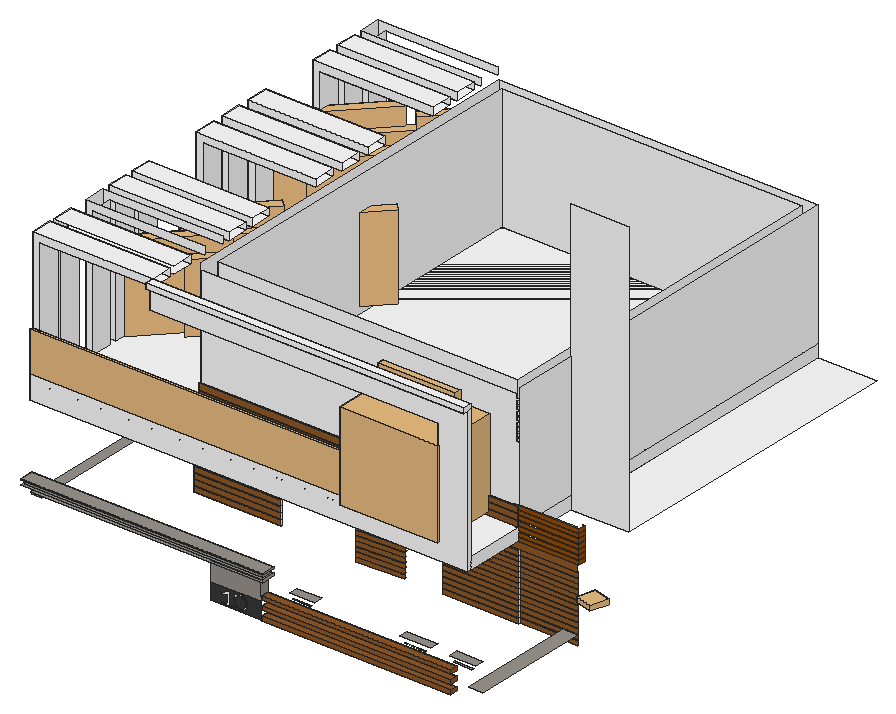
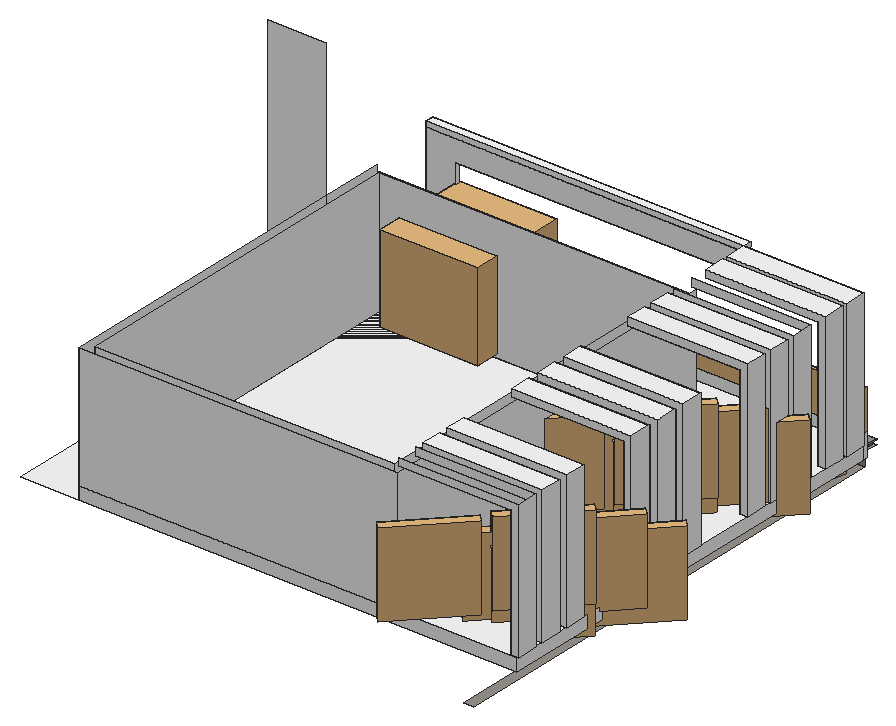
# SketchUp Ruby script. Lengths in inches.
U = 1.inch
M = Sketchup.active_model
def pt(a) = Geom::Point3d.new(a.map { |v| v * U })
def face(e, loops, mat)
  f = e.add_face(loops[0].map { |a| pt(a) })
  loops[1..].each { |l| e.add_face(l.map { |a| pt(a) }).erase! }
  f.material = f.back_material = mat if mat
  f
end
# faces: each face lists its corners as indices into pts; further lists are holes
def faces(e, pts, list, mat = nil) = list.each { |f| face(e, (f[0].is_a?(Array) ? f : [f]).map { |l| l.map { |i| pts[i] } }, mat) }
# xy, xz, yz: faces in a plane at the given z, y or x. An outline is a flat list of corners, or four numbers for a rectangle; further outlines are holes
def ring(l) = l.size == 4 ? [[l[0], l[1]], [l[2], l[1]], [l[2], l[3]], [l[0], l[3]]] : l.each_slice(2).to_a
def flat(e, list, mat, &to3) = list.each { |f| face(e, (f[0].is_a?(Array) ? f : [f]).map { |l| ring(l).map { |u, v| to3.(u, v) } }, mat) }
def xy(e, z, list, mat = nil) = flat(e, list, mat) { |x, y| [x, y, z] }
def xz(e, y, list, mat = nil) = flat(e, list, mat) { |x, z| [x, y, z] }
def yz(e, x, list, mat = nil) = flat(e, list, mat) { |y, z| [x, y, z] }
def lines(e, pts, list) = list.each { |a, b| e.add_line(pt(pts[a]), pt(pts[b])) }
# prism: a flat outline (further loops are holes) pulled along v
def prism(e, loops, v, mat = nil)
  f = face(e, loops, mat); d = Geom::Vector3d.new(v.map { |x| x * U })
  f.pushpull(f.normal.samedirection?(d) ? d.length : -d.length)
end
def box(e, o, s, mat = nil) = prism(e, [[o, [o[0] + s[0], o[1], o[2]], [o[0] + s[0], o[1] + s[1], o[2]], [o[0], o[1] + s[1], o[2]]]], [0, 0, s[2]], mat)
def at(x, y, z, deg = 0) = Geom::Transformation.translation(pt([x, y, z])) * Geom::Transformation.rotation(ORIGIN, Z_AXIS, deg.degrees)
def axes(o, x, y, z) = Geom::Transformation.new([*x, 0, *y, 0, *z, 0, *pt(o).to_a, 1])
def part(name) = M.definitions.add(name)
# library, detail: a bought-in or finely detailed component or shape, given as its bounding box
def library(name, o, s) = part(name).tap { |d| box(d.entities, o, s) }
def detail(e, o, s) = box(e.add_group.entities, o, s)
def put(e, d, t, mat = nil) = e.add_instance(d, t).tap { |i| i.material = mat if mat }
def group(e, t, mat = nil) = e.add_group.tap { |g| g.transformation = t; g.material = mat if mat }.entities
root = M.entities
M.materials.add("[Color C07]").color = [153, 76, 0]
M.materials.add("[Color M00]").color = [255, 255, 255]
M.materials.add("[Color M07]").color = [58, 58, 58]
M.materials.add("[Granite Tile]").color = [155, 148, 143]
M.materials.add("[Translucent Glass Blue]").color = [100, 149, 237]
M.materials["[Translucent Glass Blue]"].alpha = 0.5
M.materials.add("[Wood Floor Parquet]").color = [145, 89, 39]
c1 = part("Group\#32")
box(c1.entities,[0,0,0],[182.46,7.0625,3.98])
c2 = library("ruselia",[-5.83,-15.14,-32.53],[55.24,20.14,57.16])
c3 = library("CM1021-ceilingfixture-VisaLighting.dwg",[51.34,51.34,0],[17.32,17.32,4.91])
c4 = part("CM1021")
put(c4.entities,c3,at(-75.2,7.58,71.26,-15))
put(c4.entities,c3,at(67.3,7.58,71.26,-15))
put(c4.entities,c3,at(180.18,7.58,71.26,-15))
c5 = part("Group\#24")
box(c5.entities,[0,-2.3125,0],[173.47,2.3125,5.79])
c6 = library("Glass+Door+1800+x+2400",[-92.74,-2.96,0],[74.8,10.14,98.43])
c7 = part("Group\#17")
box(c7.entities,[0,-2.125,0],[58.6875,4.9375,2.3125])
c8 = library("Skt_BoxwoodBall_13",[-7.4,-7.46,-2.06],[14.58,14.83,12.98])
c9 = library("Glass railing panel",[0.75,0.33,0],[60,3.22,44.35])
xy(root,48.99,[[491.52,212.5,564.8125,213.625]],"[Color M00]")
xy(root,49.18,[[410.51,209.22,410.4,211.4,455.45,213.78,455.57,211.6]],"[Color M00]")
xy(root,52.66,[[252.1,212.375,336.02,213.625]],"[Color M00]")
xy(root,53.16,[[491.52,212.5,564.8125,213.625]],"[Color M00]")
xy(root,53.35,[[252.1,212.375,336.02,213.625]],"[Color M00]")
xy(root,53.41,[[410.51,209.22,455.57,211.6,455.45,213.78,410.4,211.4]],"[Color M00]")
xy(root,53.8,[[410.51,209.22,410.4,211.4,455.45,213.78,455.57,211.6]],"[Color M00]")
xy(root,54.18,[[491.52,212.5,564.8125,213.625]],"[Color M00]")
xy(root,58.04,[[410.51,209.22,455.57,211.6,455.45,213.78,410.4,211.4]],"[Color M00]")
xy(root,58.35,[[491.52,212.5,564.8125,213.625]],"[Color M00]")
xy(root,58.41,[[252.1,212.375,336.02,213.625]],"[Color M00]")
xy(root,58.61,[[410.51,209.22,410.4,211.4,455.45,213.78,455.57,211.6]],"[Color M00]")
xy(root,58.6875,[[607.56,99.5625,620.89,213.625]],"[Granite Tile]")
xy(root,58.91,[[252.1,212.375,336.02,213.625]],"[Color M00]")
xy(root,59.36,[[491.52,212.5,564.8125,213.625]],"[Color M00]")
xy(root,62.85,[[410.51,209.22,455.57,211.6,455.45,213.78,410.4,211.4]],"[Color M00]")
xy(root,63.24,[[410.51,209.22,410.4,211.4,455.45,213.78,455.57,211.6]],"[Color M00]")
xy(root,63.54,[[491.52,212.5,564.8125,213.625]],"[Color M00]")
xy(root,63.97,[[252.1,212.375,336.02,213.625]],"[Color M00]")
xy(root,64.36,[[491.52,212.5,564.8125,213.625]],"[Color M00]")
xy(root,64.6,[[252.1,212.375,336.02,213.625]],"[Color M00]")
xy(root,67.48,[[410.51,209.22,455.57,211.6,455.45,213.78,410.4,211.4]],"[Color M00]")
xy(root,67.93,[[410.51,209.22,410.4,211.4,455.45,213.78,455.57,211.6]],"[Color M00]")
xy(root,68.54,[[491.52,212.5,564.8125,213.625]],"[Color M00]")
xy(root,69.36,[[491.52,212.5,564.8125,213.625]],"[Color M00]")
xy(root,69.66,[[252.1,212.375,336.02,213.625]],"[Color M00]")
xy(root,70.28,[[252.1,212.375,336.02,213.625]],"[Color M00]")
xy(root,72.16,[[410.51,209.22,455.57,211.6,455.45,213.78,410.4,211.4]],"[Color M00]")
xy(root,72.78,[[410.62,209.22,410.5,211.41,455.55,213.79,455.67,211.6]],"[Color M00]")
xy(root,73.54,[[491.52,212.5,564.8125,213.625]],"[Color M00]")
xy(root,74.43,[[491.52,212.5,564.8125,213.625]],"[Color M00]")
xy(root,75.35,[[252.1,212.375,336.02,213.625]],"[Color M00]")
xy(root,75.6875,[[183.25,102.22,193.4375,573.625]],"[Granite Tile]")
xy(root,75.78,[[252.1,212.375,336.02,213.625]],"[Color M00]")
xy(root,77.01,[[410.62,209.22,455.67,211.6,455.55,213.79,410.5,211.41]],"[Color M00]")
xy(root,77.25,[[410.74,209,410.63,211.18,455.68,213.57,455.8,211.38]],"[Color M00]")
xy(root,78.6,[[491.52,212.5,564.8125,213.625]],"[Color M00]")
xy(root,79.18,[[491.52,212.5,564.8125,213.625]],"[Color M00]")
xy(root,80.75,[[551.82,91.25,572.14,91.8125]],"[Granite Tile]")
xy(root,80.85,[[252.1,212.375,336.02,213.625]],"[Color M00]")
xy(root,80.85,[[598.93,91.25,617.05,93]],"[Granite Tile]")
xy(root,80.89,[[444.42,91.25,461.86,91.8125]],"[Granite Tile]")
xy(root,81.47,[[252.1,212.375,336.02,213.625]],"[Color M00]")
xy(root,81.49,[[410.74,209,455.8,211.38,455.68,213.57,410.63,211.18]],"[Color M00]")
xy(root,81.9375,[[410.74,209,410.63,211.18,455.68,213.57,455.8,211.38]],"[Color M00]")
xy(root,83.35,[[491.52,212.5,564.8125,213.625]],"[Color M00]")
xy(root,83.93,[[491.52,212.5,564.8125,213.625]],"[Color M00]")
xy(root,85.375,[[440.87,91.25,465.26,99.5625],[547.3,91.25,577.46,99.5625],[595.47,91.25,620.89,99.5625]],"[Granite Tile]")
xy(root,86.18,[[410.74,209,455.8,211.38,455.68,213.57,410.63,211.18]],"[Color M00]")
xy(root,86.53,[[252.1,212.375,336.02,213.625]],"[Color M00]")
xy(root,86.6875,[[410.74,209,410.63,211.18,455.68,213.57,455.8,211.38]],"[Color M00]")
xy(root,86.92,[[193.4375,88.8125,417,102.22]],"[Granite Tile]")
xy(root,86.9375,[[364.82,91.25,413.01,99.5625]],"[Granite Tile]")
xy(root,87.58,[[252.1,212.375,336.02,213.625]],"[Color M00]")
xy(root,88.1,[[491.52,212.5,564.8125,213.625]],"[Color M00]")
xy(root,88.68,[[491.52,212.5,564.8125,213.625]],"[Color M00]")
xy(root,89.375,[[[183.25,88.8125,417,102.22],[185.6,91.54,415.04,100.36]]],"[Granite Tile]")
xy(root,90.93,[[410.74,209,455.8,211.38,455.68,213.57,410.63,211.18]],"[Color M00]")
xy(root,91.3125,[[410.74,209,410.63,211.18,455.68,213.57,455.8,211.38]],"[Color M00]")
xy(root,92.64,[[252.1,212.375,336.02,213.625]],"[Color M00]")
xy(root,92.85,[[491.52,212.5,564.8125,213.625]],"[Color M00]")
xy(root,93,[[183.25,88.8125,417,91.54],[183.25,91.54,185.6,102.22],[415.04,91.54,417,100.36],[185.6,100.36,417,102.22]],"[Granite Tile]")
xy(root,93.36,[[491.52,212.5,564.8125,213.625]],"[Color M00]")
xy(root,93.64,[[252.1,212.375,336.02,213.625]],"[Color M00]")
xy(root,94.5625,[[183.25,88.8125,417,102.22]],"[Granite Tile]")
xy(root,95.55,[[410.74,209,455.8,211.38,455.68,213.57,410.63,211.18]],"[Color M00]")
xy(root,96.875,[[410.74,209,410.63,211.18,455.68,213.57,455.8,211.38]],"[Color M00]")
xy(root,97.54,[[491.52,212.5,564.8125,213.625]],"[Color M00]")
xy(root,97.99,[[491.52,212.5,564.8125,213.625]],"[Color M00]")
xy(root,98.7,[[252.1,212.375,336.02,213.625]],"[Color M00]")
xy(root,99.83,[[252.1,212.375,336.02,213.625]],"[Color M00]")
xy(root,101.11,[[410.74,209,455.8,211.38,455.68,213.57,410.63,211.18]],"[Color M00]")
xy(root,102,[[410.74,209,410.63,211.18,455.68,213.57,455.8,211.38]],"[Color M00]")
xy(root,102.16,[[491.52,212.5,564.8125,213.625]],"[Color M00]")
xy(root,102.82,[[491.52,212.5,564.8125,213.625]],"[Color M00]")
xy(root,104.89,[[252.1,212.375,336.02,213.625]],"[Color M00]")
xy(root,106.14,[[252.1,212.375,336.02,213.625]],"[Color M00]")
xy(root,106.24,[[410.74,209,455.8,211.38,455.68,213.57,410.63,211.18]],"[Color M00]")
xy(root,106.875,[[410.74,209,410.63,211.18,455.68,213.57,455.8,211.38]],"[Color M00]")
xy(root,106.99,[[491.52,212.5,564.8125,213.625]],"[Color M00]")
xy(root,107.57,[[491.52,212.5,564.8125,213.625]],"[Color M00]")
xy(root,111.11,[[410.74,209,455.8,211.38,455.68,213.57,410.63,211.18]],"[Color M00]")
xy(root,111.2,[[252.1,212.375,336.02,213.625]],"[Color M00]")
xy(root,111.74,[[491.52,212.5,564.8125,213.625]],"[Color M00]")
xy(root,113.1,[[252.1,212.5,620.9375,213.625]],"[Color M00]")
xy(root,120,[[141.8125,151.875,564.8125,155.5],[252.1,212.5,620.9375,213.625],[564.8125,275.23,620.9375,573.625]],"[Color M00]")
xy(root,120.2,[[561.375,211.8125,561.375,213.625,622.25,213.625,622.25,218.625,623.5625,218.625,623.5625,211.8125]],"[Color M00]")
xy(root,123.76,[[561.375,211.8125,623.5625,211.8125,623.5625,218.625,622.25,218.625,622.25,213.625,561.375,213.625]],"[Color M00]")
xy(root,124.89,[[561.375,211.8125,561.375,213.625,622.25,213.625,622.25,218.625,623.5625,218.625,623.5625,211.8125]],"[Color M00]")
xy(root,128.45,[[561.375,211.8125,623.5625,211.8125,623.5625,218.625,622.25,218.625,622.25,213.625,561.375,213.625]],"[Color M00]")
xy(root,129.65,[[561.375,211.8125,561.375,213.625,622.25,213.625,622.25,218.625,623.5625,218.625,623.5625,211.8125]],"[Color M00]")
xy(root,132,[[[257.3125,213.625,564.8125,573.625],[266.75,222.625,555.8125,564.625]],[141.8125,219.03,149.03,239.92],[266.75,222.625,555.8125,564.625]],"[Color M00]")
xy(root,133.21,[[561.375,211.8125,623.5625,211.8125,623.5625,218.625,622.25,218.625,622.25,213.625,561.375,213.625]],"[Color M00]")
xy(root,134.4,[[561.375,211.8125,561.375,213.625,622.25,213.625,622.25,218.625,623.5625,218.625,623.5625,211.8125]],"[Color M00]")
xy(root,137.96,[[561.375,211.8125,623.5625,211.8125,623.5625,218.625,622.25,218.625,622.25,213.625,561.375,213.625]],"[Color M00]")
xy(root,139.15,[[561.375,211.8125,561.375,213.625,622.25,213.625,622.25,218.625,623.5625,218.625,623.5625,211.8125]],"[Color M00]")
xy(root,142.37,[[141.8125,151.875,535.19,155.5]],"[Color M00]")
xy(root,142.71,[[561.375,211.8125,623.5625,211.8125,623.5625,218.625,622.25,218.625,622.25,213.625,561.375,213.625]],"[Color M00]")
xy(root,143.59,[[561.375,211.8125,561.375,213.625,622.25,213.625,622.25,218.625,623.5625,218.625,623.5625,211.8125]],"[Color M00]")
xy(root,147.15,[[561.375,211.8125,623.5625,211.8125,623.5625,218.625,622.25,218.625,622.25,213.625,561.375,213.625]],"[Color M00]")
xy(root,147.77,[[561.375,211.8125,561.375,213.625,622.25,213.625,622.25,218.625,623.5625,218.625,623.5625,211.8125]],"[Color M00]")
xy(root,238.5625,[[257.3125,151.875,535.19,155.5]],"[Color M00]")
xy(root,256.75,[[149.03,155.5,257.3125,176.39],[149.03,180.8125,257.3125,201.7],[149.03,247.28,257.3125,268.17],[149.03,274.72,257.3125,295.61],[149.03,352.5625,257.3125,373.45],
  [149.03,383.5,257.3125,404.39],[149.03,415.3125,257.3125,436.2],[149.03,492.9375,257.3125,513.83],[149.03,522.625,257.3125,543.51]],"[Color M00]")
xy(root,259.26,[[257.3125,146.9375,564.8125,151.875],[257.3125,151.875,564.8125,155.5]],"[Color M00]")
xy(root,264,[[257.3125,146.9375,564.8125,155.5],[141.8125,155.5,257.3125,176.39],[141.8125,180.8125,257.3125,201.7],[141.8125,247.28,257.3125,268.17],[141.8125,274.72,257.3125,295.61],
  [141.8125,352.5625,257.3125,373.45],[141.8125,383.5,257.3125,404.39],[141.8125,415.3125,257.3125,436.2],[141.8125,492.9375,257.3125,513.83],[141.8125,522.625,257.3125,543.51]],"[Color M00]")
xz(root,88.8125,[[183.25,93,417,94.5625]],"[Granite Tile]")
xz(root,91.25,[[[393.28,53.49,395.01,53.64,396.63,54.23,398.05,55.22,399.16,56.54,399.9,58.11,400.2,59.81,400.05,61.53,399.47,63.16,398.48,64.58,397.15,65.69,395.59,66.43,393.89,66.73,392.16,66.58,390.54,65.99,389.12,65,388,63.68,387.27,62.12,386.97,60.41,387.11,58.69,387.7,57.0625,388.69,55.64,390.01,54.53,391.58,53.8],[393.58,54.86,392.23,55.04,390.96,55.5625,389.87,56.4,389.04,57.49,388.51,58.75,388.33,60.11,388.51,61.47,389.04,62.74,389.87,63.82,390.96,64.66,392.23,65.18,393.58,65.36,394.94,65.18,396.21,64.66,397.3,63.82,398.13,62.74,398.66,61.47,398.83,60.11,398.66,58.75,398.13,57.49,397.3,56.4,396.21,55.5625,394.94,55.04]],[375.79,53.62,387.87,53.62,387.87,54.43,382.16,54.43,382.16,66.03,375.79,62.58,376.9,61.57,380.9375,63.7,380.9375,54.43,375.79,54.43]],"[Color M00]")
xz(root,91.25,[[[364.82,52.49,413.01,68.13],[393.28,53.49,391.58,53.8,390.01,54.53,388.69,55.64,387.7,57.0625,387.11,58.69,386.97,60.41,387.27,62.12,388,63.68,389.12,65,390.54,65.99,392.16,66.58,393.89,66.73,395.59,66.43,397.15,65.69,398.48,64.58,399.47,63.16,400.05,61.53,400.2,59.81,399.9,58.11,399.16,56.54,398.05,55.22,396.63,54.23,395.01,53.64],[375.79,53.62,375.79,54.43,380.9375,54.43,380.9375,63.7,376.9,61.57,375.79,62.58,382.16,66.03,382.16,54.43,387.87,54.43,387.87,53.62]],[393.58,54.86,394.94,55.04,396.21,55.5625,397.3,56.4,398.13,57.49,398.66,58.75,398.83,60.11,398.66,61.47,398.13,62.74,397.3,63.82,396.21,64.66,394.94,65.18,393.58,65.36,392.23,65.18,390.96,64.66,389.87,63.82,389.04,62.74,388.51,61.47,388.33,60.11,388.51,58.75,389.04,57.49,389.87,56.4,390.96,55.5625,392.23,55.04]],"[Color M07]")
xz(root,91.25,[[364.82,68.13,413.01,86.9375]],"[Granite Tile]")
xz(root,91.54,[[185.6,89.375,415.04,93]],"[Granite Tile]")
xz(root,100.36,[[185.6,89.375,415.04,93]],"[Granite Tile]")
xz(root,102.22,[[183.25,75.6875,193.4375,75.6875,193.4375,86.92,417,86.92,417,89.375,183.25,89.375],[183.25,93,417,94.5625]],"[Granite Tile]")
xz(root,146.9375,[[257.3125,259.26,564.8125,264]],"[Color M00]")
xz(root,151.875,[[141.8125,120,564.8125,120,564.8125,259.26,257.3125,259.26,257.3125,238.5625,535.19,238.5625,535.19,142.37,141.8125,142.37]],"[Color M00]")
xz(root,155.5,[[141.8125,120,141.8125,132,149.03,132,149.03,142.37,535.19,142.37,535.19,238.5625,257.3125,238.5625,257.3125,259.26,564.8125,259.26,564.8125,120],[141.8125,132,149.03,142.37],[141.8125,142.37,149.03,142.37,149.03,256.75,257.3125,256.75,257.3125,264,141.8125,264],[257.3125,259.26,564.8125,264]],"[Color M00]")
xz(root,176.39,[[141.8125,132,141.8125,264,257.3125,264,257.3125,256.75,149.03,256.75,149.03,132]],"[Color M00]")
xz(root,180.8125,[[141.8125,132,149.03,142.37]],"[Color M00]")
xz(root,201.7,[[141.8125,132,141.8125,264,257.3125,264,257.3125,256.75,149.03,256.75,149.03,132]],"[Color M00]")
xz(root,211.8125,[[561.375,120.2,623.5625,123.76],[561.375,124.89,623.5625,128.45],[561.375,129.65,623.5625,133.21],[561.375,134.4,623.5625,137.96],[561.375,139.15,623.5625,142.71],
  [561.375,143.59,623.5625,147.15],[561.375,147.77,623.5625,151.34]],"[Color C07]")
xz(root,212.375,[[252.1,53.35,336.02,58.41],[252.1,58.91,336.02,63.97],[252.1,64.6,336.02,69.66],[252.1,70.28,336.02,75.35],[252.1,75.78,336.02,80.85],
  [252.1,81.47,336.02,86.53],[252.1,87.58,336.02,92.64],[252.1,93.64,336.02,98.7],[252.1,99.83,336.02,104.89],[252.1,106.14,336.02,111.2]],"[Wood Floor Parquet]")
xz(root,212.5,[[491.52,48.99,564.8125,53.16],[491.52,54.18,564.8125,58.35],[491.52,59.36,564.8125,63.54],[491.52,64.36,564.8125,68.54],[491.52,69.36,564.8125,73.54],
  [491.52,74.43,564.8125,78.6],[491.52,79.18,564.8125,83.35],[491.52,83.93,564.8125,88.1],[491.52,88.68,564.8125,92.85],[491.52,93.36,564.8125,97.54],
  [491.52,97.99,564.8125,102.16],[491.52,102.82,564.8125,106.99],[491.52,107.57,564.8125,111.74],[252.1,113.1,620.9375,120]],"[Wood Floor Parquet]")
xz(root,213.625,[[252.1,53.35,336.02,58.41],[252.1,58.91,336.02,63.97],[252.1,64.6,336.02,69.66],[252.1,70.28,336.02,75.35],[252.1,75.78,336.02,80.85],
  [252.1,81.47,336.02,86.53],[252.1,87.58,336.02,92.64],[252.1,93.64,336.02,98.7],[252.1,99.83,336.02,104.89],[252.1,106.14,336.02,111.2],
  [491.52,107.57,564.8125,111.74],[257.3125,132,564.8125,132,564.8125,204.71,561.375,204.71,561.375,208.27,564.8125,208.27,564.8125,209.21,561.375,209.21,561.375,212.77,564.8125,212.77,564.8125,213.84,561.375,213.84,561.375,217.4,564.8125,217.4,564.8125,218.15,561.375,218.15,561.375,221.71,564.8125,221.71,564.8125,222.96,561.375,222.96,561.375,226.52,564.8125,226.52,564.8125,227.46,561.375,227.46,561.375,231.02,564.8125,231.02,564.8125,232.46,561.375,232.46,561.375,236.02,564.8125,236.02,564.8125,237.27,561.375,237.27,561.375,240.84,564.8125,240.84,564.8125,242.46,561.375,242.46,561.375,246.02,564.8125,246.02,564.8125,246.21,257.3125,246.21]],"[Color M00]")
xz(root,213.625,[[607.56,58.35,620.89,58.6875]],"[Granite Tile]")
xz(root,213.625,[[564.8125,120,620.9375,120.2],[564.8125,120.2,620.9375,123.76],[564.8125,123.76,620.9375,124.89],[564.8125,124.89,620.9375,128.45],[564.8125,128.45,620.9375,129.65],
  [564.8125,129.65,620.9375,133.21],[564.8125,133.21,620.9375,134.4],[564.8125,134.4,620.9375,137.96],[564.8125,137.96,620.9375,139.15],[564.8125,139.15,620.9375,142.71],
  [564.8125,142.71,620.9375,143.59],[564.8125,143.59,620.9375,147.15],[564.8125,147.15,620.9375,147.77],[564.8125,147.77,620.9375,151.34]],"[Translucent Glass Blue]")
xz(root,213.625,[[564.8125,48.99,607.56,53.16],[607.56,48.99,620.89,53.16],[620.89,48.99,620.9375,53.16],[607.56,53.16,620.89,54.18],[620.89,53.16,620.9375,54.18],
  [564.8125,54.18,607.56,58.35],[607.56,54.18,620.89,58.35],[620.89,54.18,620.9375,58.35],[564.8125,59.36,620.9375,63.54],[564.8125,64.36,620.9375,68.54],
  [564.8125,69.36,620.9375,73.54],[564.8125,74.43,620.9375,78.6],[564.8125,79.18,620.9375,83.35],[564.8125,83.93,620.9375,88.1],[564.8125,88.68,620.9375,92.85],
  [564.8125,93.36,620.9375,97.54],[564.8125,97.99,620.9375,102.16],[564.8125,102.82,620.9375,106.99],[564.8125,107.57,620.9375,111.74]],"[Wood Floor Parquet]")
xz(root,218.625,[[622.25,120.2,623.5625,123.76],[622.25,124.89,623.5625,128.45],[622.25,129.65,623.5625,133.21],[622.25,134.4,623.5625,137.96],[622.25,139.15,623.5625,142.71],
  [622.25,143.59,623.5625,147.15],[622.25,147.77,623.5625,151.34]],"[Color M00]")
xz(root,219.03,[[141.8125,132,149.03,132,149.03,256.75,257.3125,256.75,257.3125,264,141.8125,264]],"[Color M00]")
xz(root,222.625,[[266.75,132,555.8125,252]],"[Color M00]")
xz(root,239.92,[[141.8125,132,141.8125,264,257.3125,264,257.3125,256.75,149.03,256.75,149.03,132]],"[Color M00]")
xz(root,247.28,[[141.8125,132,149.03,132,149.03,256.75,257.3125,256.75,257.3125,264,141.8125,264]],"[Color M00]")
xz(root,268.17,[[141.8125,132,141.8125,264,257.3125,264,257.3125,256.75,149.03,256.75,149.03,132]],"[Color M00]")
xz(root,274.72,[[141.8125,132,149.03,132,149.03,256.75,257.3125,256.75,257.3125,264,141.8125,264]],"[Color M00]")
xz(root,275.23,[[564.8125,120,620.9375,384]],"[Color M00]")
xz(root,295.61,[[141.8125,132,141.8125,264,257.3125,264,257.3125,256.75,149.03,256.75,149.03,132]],"[Color M00]")
xz(root,352.5625,[[141.8125,132,149.03,132,149.03,256.75,257.3125,256.75,257.3125,264,141.8125,264]],"[Color M00]")
xz(root,373.45,[[141.8125,132,141.8125,264,257.3125,264,257.3125,256.75,149.03,256.75,149.03,132]],"[Color M00]")
xz(root,383.5,[[141.8125,132,149.03,132,149.03,256.75,257.3125,256.75,257.3125,264,141.8125,264]],"[Color M00]")
xz(root,404.39,[[141.8125,132,141.8125,264,257.3125,264,257.3125,256.75,149.03,256.75,149.03,132]],"[Color M00]")
xz(root,415.3125,[[141.8125,132,149.03,132,149.03,256.75,257.3125,256.75,257.3125,264,141.8125,264]],"[Color M00]")
xz(root,436.2,[[141.8125,132,141.8125,264,257.3125,264,257.3125,256.75,149.03,256.75,149.03,132]],"[Color M00]")
xz(root,492.9375,[[141.8125,132,149.03,132,149.03,256.75,257.3125,256.75,257.3125,264,141.8125,264]],"[Color M00]")
xz(root,513.83,[[141.8125,132,141.8125,264,257.3125,264,257.3125,256.75,149.03,256.75,149.03,132]],"[Color M00]")
xz(root,522.625,[[141.8125,132,149.03,132,149.03,256.75,257.3125,256.75,257.3125,264,141.8125,264]],"[Color M00]")
xz(root,543.51,[[141.8125,132,141.8125,264,257.3125,264,257.3125,256.75,149.03,256.75,149.03,132]],"[Color M00]")
xz(root,551.125,[[141.8125,132,149.03,132,149.03,256.75,257.3125,256.75,257.3125,264,141.8125,264]],"[Color M00]")
xz(root,564.625,[[266.75,132,555.8125,252]],"[Color M00]")
xz(root,572.01,[[141.8125,132,141.8125,264,257.3125,264,257.3125,256.75,149.03,256.75,149.03,132]],"[Color M00]")
xz(root,573.625,[[257.3125,132,564.8125,252]],"[Color M00]")
yz(root,141.8125,[[151.875,120,155.5,142.37],[155.5,132,176.39,264],[180.8125,132,201.7,264],[219.03,132,239.92,264],[247.28,132,268.17,264],
  [274.72,132,295.61,264],[352.5625,132,373.45,264],[383.5,132,404.39,264],[415.3125,132,436.2,264],[492.9375,132,513.83,264],
  [522.625,132,543.51,264],[551.125,132,572.01,264]],"[Color M00]")
yz(root,149.03,[[155.5,132,176.39,256.75],[180.8125,132,201.7,256.75],[219.03,132,239.92,256.75],[247.28,132,268.17,256.75],[274.72,132,295.61,256.75],
  [352.5625,132,373.45,256.75],[383.5,132,404.39,256.75],[415.3125,132,436.2,256.75],[492.9375,132,513.83,256.75],[522.625,132,543.51,256.75],
  [551.125,132,572.01,256.75]],"[Color M00]")
yz(root,183.25,[[88.8125,93,102.22,94.5625]],"[Granite Tile]")
yz(root,185.6,[[91.54,89.375,100.36,93]],"[Granite Tile]")
yz(root,252.1,[[212.375,53.35,213.625,58.41],[212.375,58.91,213.625,63.97],[212.375,64.6,213.625,69.66],[212.375,70.28,213.625,75.35],[212.375,75.78,213.625,80.85],
  [212.375,81.47,213.625,86.53],[212.375,87.58,213.625,92.64],[212.375,93.64,213.625,98.7],[212.375,99.83,213.625,104.89],[212.375,106.14,213.625,111.2]],"[Color M00]")
yz(root,257.3125,[[213.625,132,573.625,252],[151.875,238.5625,155.5,259.26],[146.9375,259.26,155.5,264]],"[Color M00]")
yz(root,266.75,[[222.625,132,564.625,252]],"[Color M00]")
yz(root,336.02,[[212.375,53.35,213.625,58.41],[212.375,58.91,213.625,63.97],[212.375,64.6,213.625,69.66],[212.375,70.28,213.625,75.35],[212.375,75.78,213.625,80.85],
  [212.375,81.47,213.625,86.53],[212.375,87.58,213.625,92.64],[212.375,93.64,213.625,98.7],[212.375,99.83,213.625,104.89],[212.375,106.14,213.625,111.2]],"[Color M00]")
yz(root,413.01,[[91.25,72.61,99.5625,86.9375]],"[Granite Tile]")
yz(root,415.04,[[91.54,89.375,100.36,93]],"[Granite Tile]")
yz(root,417,[[88.8125,86.92,102.22,89.375],[88.8125,93,102.22,94.5625]],"[Granite Tile]")
yz(root,491.52,[[212.5,107.57,213.625,111.74]],"[Color M00]")
yz(root,535.19,[[151.875,142.37,155.5,238.5625]],"[Color M00]")
yz(root,555.8125,[[222.625,132,564.625,252]],"[Color M00]")
yz(root,564.8125,[[212.5,48.99,213.625,53.16],[212.5,54.18,213.625,58.35],[212.5,59.36,213.625,63.54],[212.5,64.36,213.625,68.54],[212.5,69.36,213.625,73.54],
  [212.5,74.43,213.625,78.6],[212.5,79.18,213.625,83.35],[212.5,83.93,213.625,88.1],[212.5,88.68,213.625,92.85],[212.5,93.36,213.625,97.54],
  [212.5,97.99,213.625,102.16],[212.5,102.82,213.625,106.99],[212.5,107.57,213.625,111.74],[151.875,120,155.5,259.26],[213.625,120,275.23,132],
  [213.625,132,275.23,252],[275.23,132,573.625,252],[146.9375,259.26,155.5,264]],"[Color M00]")
yz(root,623.5625,[[211.8125,120.2,218.625,123.76],[211.8125,124.89,218.625,128.45],[211.8125,129.65,218.625,133.21],[211.8125,134.4,218.625,137.96],[211.8125,139.15,218.625,142.71],
  [211.8125,143.59,218.625,147.15],[211.8125,147.77,218.625,151.34]],"[Color C07]")
p = [[410.51,209.22,49.18],[455.57,211.6,49.18],[455.57,211.6,53.41],[410.51,209.22,53.41],[410.51,209.22,53.8],[455.57,211.6,53.8],
  [455.57,211.6,58.04],[410.51,209.22,58.04],[410.51,209.22,58.61],[455.57,211.6,58.61],[455.57,211.6,62.85],[410.51,209.22,62.85],
  [410.51,209.22,63.24],[455.57,211.6,63.24],[455.57,211.6,67.48],[410.51,209.22,67.48],[410.51,209.22,67.93],[455.57,211.6,67.93],
  [455.57,211.6,72.16],[410.51,209.22,72.16],[410.62,209.22,72.78],[455.67,211.6,72.78],[455.67,211.6,77.01],[410.62,209.22,77.01],
  [410.74,209,77.25],[455.8,211.38,77.25],[455.8,211.38,81.49],[410.74,209,81.49],[410.74,209,81.9375],[455.8,211.38,81.9375],
  [455.8,211.38,86.18],[410.74,209,86.18],[410.74,209,86.6875],[455.8,211.38,86.6875],[455.8,211.38,90.93],[410.74,209,90.93],
  [410.74,209,91.3125],[455.8,211.38,91.3125],[455.8,211.38,95.55],[410.74,209,95.55],[410.74,209,96.875],[455.8,211.38,96.875],
  [455.8,211.38,101.11],[410.74,209,101.11],[410.74,209,102],[455.8,211.38,102],[455.8,211.38,106.24],[410.74,209,106.24],
  [410.63,211.18,111.11],[410.63,211.18,106.875],[410.74,209,106.875],[410.74,209,111.11],[455.8,211.38,106.875],[455.8,211.38,111.11],
  [455.68,213.57,106.875],[455.68,213.57,111.11]]
faces(root,p,[[0,1,2,3],[4,5,6,7],[8,9,10,11],[12,13,14,15],[16,17,18,19],[20,21,22,23],[24,25,26,27],[28,29,30,31],
  [32,33,34,35],[36,37,38,39],[40,41,42,43],[44,45,46,47],[50,52,53,51]],"[Wood Floor Parquet]")
faces(root,p,[[48,49,50,51],[54,49,48,55],[54,55,53,52]],"[Color M00]")
put(root,c1,at(413.01,92.5,50.94),"[Wood Floor Parquet]")
put(root,c1,at(413.01,92.5,59.75),"[Wood Floor Parquet]")
put(root,c1,at(413.01,92.5,68.63),"[Wood Floor Parquet]")
put(root,c2,axes([201.14,521.4,160.65],[-0.97449,-1.03284,0],[1.03284,-0.97449,0],[0,0,1.42]),"[Granite Tile]")
put(root,c4,at(156.5625,130.16,43.37),"[Granite Tile]")
put(root,c4,at(408.25,130.16,43.37),"[Granite Tile]")
put(root,c2,axes([150.39,470.56,161.26],[-0.97449,-1.03284,0],[0.34084,-0.32158,0],[0,0,1.42]),"[Granite Tile]")
put(root,c2,axes([228.2,340.45,163.29],[-0.97449,-1.03284,0],[1.03284,-0.97449,0],[0,0,1.42]),"[Granite Tile]")
put(root,c2,axes([177.44,289.61,163.89],[-0.97449,-1.03284,0],[0.34084,-0.32158,0],[0,0,1.42]),"[Granite Tile]")
g1 = group(root,at(204.8125,573.625,120),"[Color M00]")
box(g1,[-63,-418.125,0],[423,418.125,12])
put(root,c2,axes([209.47,543.45,172.26],[-0.97449,-1.03284,0],[0.34084,-0.32158,0],[0,0,1.42]),"[Granite Tile]")
put(root,c2,axes([236.53,362.5,174.9],[-0.97449,-1.03284,0],[0.34084,-0.32158,0],[0,0,1.42]),"[Granite Tile]")
put(root,c2,axes([169.84,494.9,175.4],[-0.97449,-1.03284,0],[0.34084,-0.32158,0],[0,0,1.42]),"[Granite Tile]")
put(root,c5,at(257.3125,213.625,129.41),"[Wood Floor Parquet]")
put(root,c2,axes([196.89,313.95,178.04],[-0.97449,-1.03284,0],[0.34084,-0.32158,0],[0,0,1.42]),"[Granite Tile]")
put(root,c6,at(526,209.75,132),"[Color M00]")
put(root,c7,axes([506.125,213.625,135.33],[1,0,0],[0,0,1],[0,-1,0]),"[Wood Floor Parquet]")
put(root,c8,axes([489.85,198.66,149.33],[6.4872,0,0],[0,6.4872,0],[0,0,6.4872]),"[Granite Tile]")
put(root,c5,at(257.3125,213.625,136.5625),"[Wood Floor Parquet]")
put(root,c2,axes([252.62,591.11,182.85],[-0.97449,-1.03284,0],[0.34084,-0.32158,0],[0,0,1.42]),"[Granite Tile]")
put(root,c9,axes([137.11,151.875,136.87],[6.5528,0,0],[0,1,0],[0,0,1]),"[Color M00]")
put(root,c7,axes([506.125,213.625,141.39],[1,0,0],[0,0,1],[0,-1,0]),"[Wood Floor Parquet]")
put(root,c2,axes([279.68,410.16,185.48],[-0.97449,-1.03284,0],[0.34084,-0.32158,0],[0,0,1.42]),"[Granite Tile]")
put(root,c2,axes([188.54,532.96,189.22],[-0.97449,-1.03284,0],[0.34084,-0.32158,0],[0,0,1.42]),"[Granite Tile]")
put(root,c5,at(257.3125,213.625,143.25),"[Wood Floor Parquet]")
put(root,c7,axes([506.125,213.625,147.14],[1,0,0],[0,0,1],[0,-1,0]),"[Wood Floor Parquet]")
put(root,c2,axes([215.6,352.01,191.86],[-0.97449,-1.03284,0],[0.34084,-0.32158,0],[0,0,1.42]),"[Granite Tile]")
